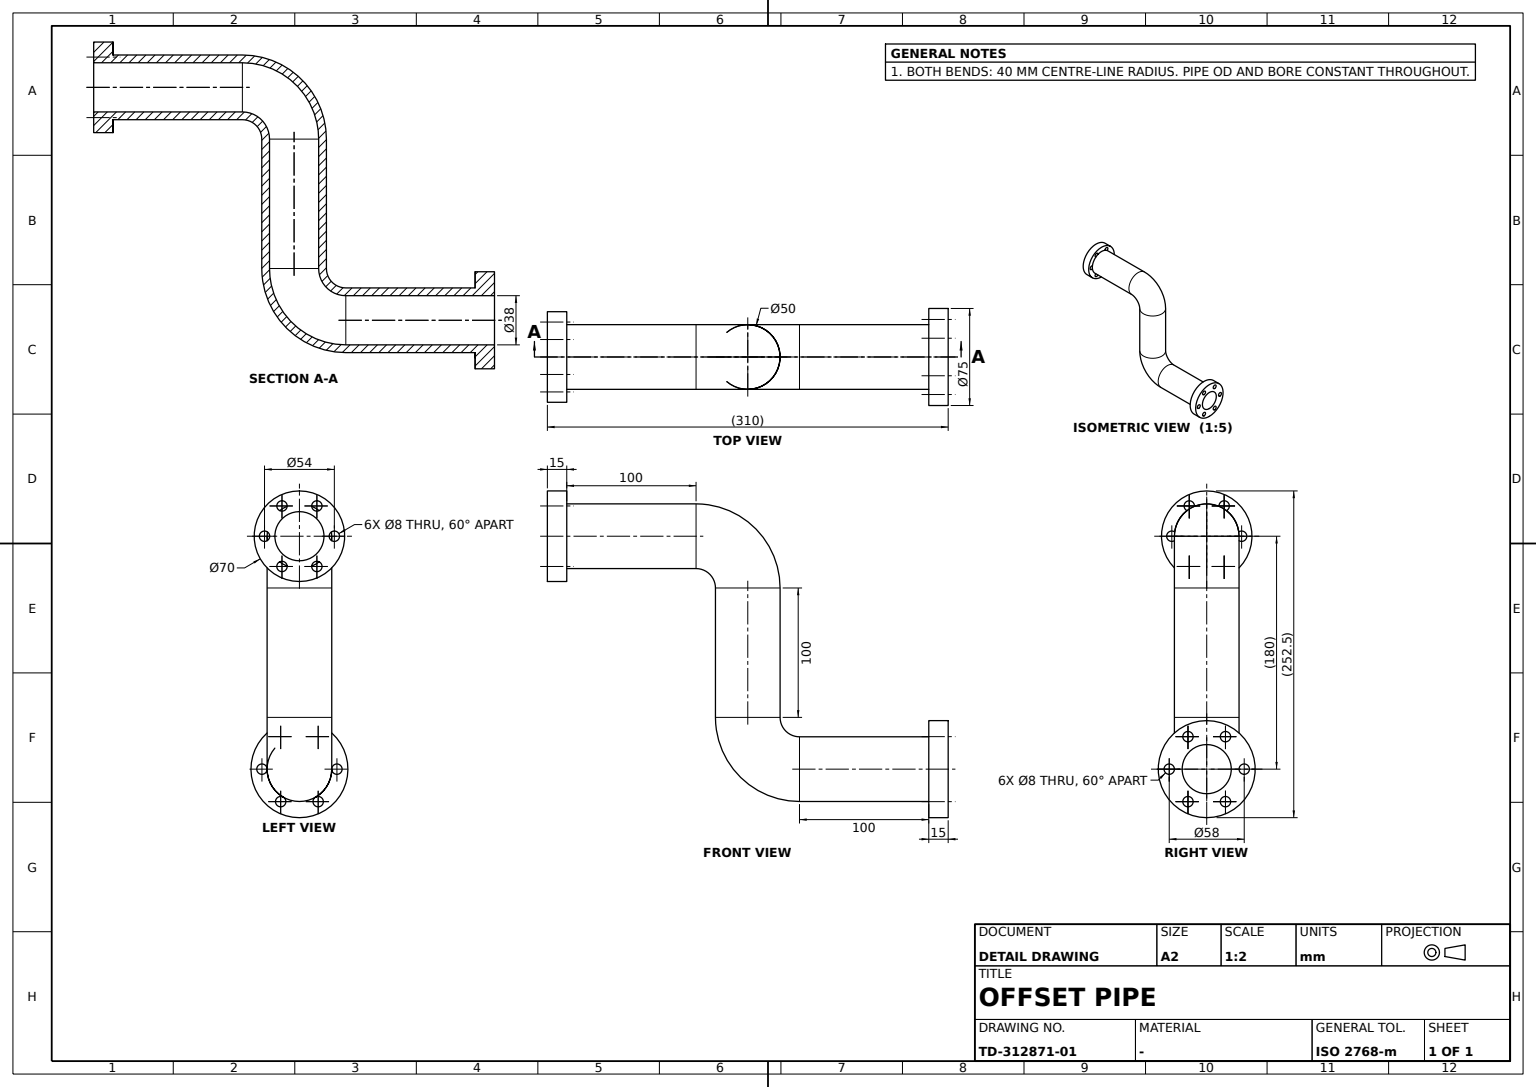
ISO-10303-21;
HEADER;
FILE_DESCRIPTION((''),'2;1');
FILE_NAME('','',(''),(''),'','','');
FILE_SCHEMA(('AUTOMOTIVE_DESIGN'));
ENDSEC;
DATA;
#1=APPLICATION_CONTEXT('');
#2=PRODUCT_CONTEXT('',#1,'mechanical');
#3=PRODUCT('','','',(#2));
#4=PRODUCT_DEFINITION_FORMATION('','',#3);
#5=PRODUCT_DEFINITION_CONTEXT('',#1,'design');
#6=PRODUCT_DEFINITION('','',#4,#5);
#7=PRODUCT_DEFINITION_SHAPE('','',#6);
#8=(LENGTH_UNIT()NAMED_UNIT(*)SI_UNIT(.MILLI.,.METRE.));
#9=(NAMED_UNIT(*)PLANE_ANGLE_UNIT()SI_UNIT($,.RADIAN.));
#10=(NAMED_UNIT(*)SI_UNIT($,.STERADIAN.)SOLID_ANGLE_UNIT());
#11=UNCERTAINTY_MEASURE_WITH_UNIT(LENGTH_MEASURE(0.005),#8,'distance_accuracy_value','');
#12=(GEOMETRIC_REPRESENTATION_CONTEXT(3)GLOBAL_UNCERTAINTY_ASSIGNED_CONTEXT((#11))GLOBAL_UNIT_ASSIGNED_CONTEXT((#8,#9,#10))REPRESENTATION_CONTEXT('',''));
#13=CARTESIAN_POINT('',(-165.,0.,40.));
#14=VERTEX_POINT('',#13);
#15=CARTESIAN_POINT('',(-140.,0.,40.));
#16=DIRECTION('',(0.,0.,-1.));
#17=DIRECTION('',(-1.,0.,0.));
#18=AXIS2_PLACEMENT_3D('',#15,#16,#17);
#19=CIRCLE('',#18,25.);
#20=EDGE_CURVE('',#14,#14,#19,.T.);
#21=ORIENTED_EDGE('',*,*,#20,.F.);
#22=EDGE_LOOP('',(#21));
#23=FACE_BOUND('',#22,.T.);
#24=CARTESIAN_POINT('',(-165.,0.,140.));
#25=VERTEX_POINT('',#24);
#26=CARTESIAN_POINT('',(-140.,0.,140.));
#27=AXIS2_PLACEMENT_3D('',#26,#16,#17);
#28=CIRCLE('',#27,25.);
#29=EDGE_CURVE('',#25,#25,#28,.T.);
#30=ORIENTED_EDGE('',*,*,#29,.T.);
#31=EDGE_LOOP('',(#30));
#32=FACE_BOUND('',#31,.T.);
#33=CARTESIAN_POINT('',(-140.,0.,90.));
#34=DIRECTION('',(0.,1.,0.));
#35=AXIS2_PLACEMENT_3D('',#33,#16,#34);
#36=CYLINDRICAL_SURFACE('',#35,25.);
#37=ADVANCED_FACE('',(#23,#32),#36,.T.);
#38=CARTESIAN_POINT('',(0.,-25.,0.));
#39=VERTEX_POINT('',#38);
#40=CARTESIAN_POINT('',(0.,-29.,0.));
#41=DIRECTION('',(1.,0.,0.));
#42=AXIS2_PLACEMENT_3D('',#40,#41,#16);
#43=CIRCLE('',#42,4.);
#44=EDGE_CURVE('',#39,#39,#43,.T.);
#45=ORIENTED_EDGE('',*,*,#44,.F.);
#46=EDGE_LOOP('',(#45));
#47=FACE_BOUND('',#46,.T.);
#48=CARTESIAN_POINT('',(15.,-29.,-4.));
#49=VERTEX_POINT('',#48);
#50=CARTESIAN_POINT('',(15.,-29.,0.));
#51=AXIS2_PLACEMENT_3D('',#50,#41,#16);
#52=CIRCLE('',#51,4.);
#53=EDGE_CURVE('',#49,#49,#52,.T.);
#54=ORIENTED_EDGE('',*,*,#53,.T.);
#55=EDGE_LOOP('',(#54));
#56=FACE_BOUND('',#55,.T.);
#57=CARTESIAN_POINT('',(7.5,-29.,0.));
#58=DIRECTION('',(0.,-1.,0.));
#59=AXIS2_PLACEMENT_3D('',#57,#41,#58);
#60=CYLINDRICAL_SURFACE('',#59,4.);
#61=ADVANCED_FACE('',(#47,#56),#60,.F.);
#62=CARTESIAN_POINT('',(15.,14.5,21.114737));
#63=VERTEX_POINT('',#62);
#64=CARTESIAN_POINT('',(15.,14.5,25.114737));
#65=AXIS2_PLACEMENT_3D('',#64,#41,#16);
#66=CIRCLE('',#65,4.);
#67=EDGE_CURVE('',#63,#63,#66,.T.);
#68=ORIENTED_EDGE('',*,*,#67,.T.);
#69=EDGE_LOOP('',(#68));
#70=FACE_BOUND('',#69,.T.);
#71=CARTESIAN_POINT('',(0.,12.5,21.650635));
#72=VERTEX_POINT('',#71);
#73=CARTESIAN_POINT('',(0.,14.5,25.114737));
#74=AXIS2_PLACEMENT_3D('',#73,#41,#16);
#75=CIRCLE('',#74,4.);
#76=EDGE_CURVE('',#72,#72,#75,.T.);
#77=ORIENTED_EDGE('',*,*,#76,.F.);
#78=EDGE_LOOP('',(#77));
#79=FACE_BOUND('',#78,.T.);
#80=CARTESIAN_POINT('',(7.5,14.5,25.114737));
#81=DIRECTION('',(0.,0.5,0.866025404));
#82=AXIS2_PLACEMENT_3D('',#80,#41,#81);
#83=CYLINDRICAL_SURFACE('',#82,4.);
#84=ADVANCED_FACE('',(#70,#79),#83,.F.);
#85=CARTESIAN_POINT('',(-180.,0.,199.));
#86=VERTEX_POINT('',#85);
#87=CARTESIAN_POINT('',(-180.,0.,180.));
#88=DIRECTION('',(0.,0.,1.));
#89=AXIS2_PLACEMENT_3D('',#87,#17,#88);
#90=CIRCLE('',#89,19.);
#91=EDGE_CURVE('',#86,#86,#90,.F.);
#92=ORIENTED_EDGE('',*,*,#91,.T.);
#93=EDGE_LOOP('',(#92));
#94=FACE_BOUND('',#93,.T.);
#95=CARTESIAN_POINT('',(-295.,0.,199.));
#96=VERTEX_POINT('',#95);
#97=CARTESIAN_POINT('',(-295.,0.,180.));
#98=AXIS2_PLACEMENT_3D('',#97,#17,#88);
#99=CIRCLE('',#98,19.);
#100=EDGE_CURVE('',#96,#96,#99,.T.);
#101=ORIENTED_EDGE('',*,*,#100,.T.);
#102=EDGE_LOOP('',(#101));
#103=FACE_BOUND('',#102,.T.);
#104=CARTESIAN_POINT('',(-287.5,0.,180.));
#105=AXIS2_PLACEMENT_3D('',#104,#17,#58);
#106=CYLINDRICAL_SURFACE('',#105,19.);
#107=ADVANCED_FACE('',(#94,#103),#106,.F.);
#108=CARTESIAN_POINT('',(-280.,24.777778,176.674082));
#109=VERTEX_POINT('',#108);
#110=CARTESIAN_POINT('',(-280.,24.777778,183.325918));
#111=VERTEX_POINT('',#110);
#112=CARTESIAN_POINT('',(-280.,0.,180.));
#113=AXIS2_PLACEMENT_3D('',#112,#41,#16);
#114=CIRCLE('',#113,25.);
#115=EDGE_CURVE('',#109,#111,#114,.T.);
#116=ORIENTED_EDGE('',*,*,#115,.F.);
#117=CARTESIAN_POINT('',(-280.,27.,180.));
#118=AXIS2_PLACEMENT_3D('',#117,#41,#16);
#119=CIRCLE('',#118,4.);
#120=EDGE_CURVE('',#109,#111,#119,.F.);
#121=ORIENTED_EDGE('',*,*,#120,.T.);
#122=EDGE_LOOP('',(#116,#121));
#123=FACE_BOUND('',#122,.T.);
#124=AXIS2_PLACEMENT_3D('',#112,#41,#34);
#125=PLANE('',#124);
#126=ADVANCED_FACE('',(#123),#125,.F.);
#127=CARTESIAN_POINT('',(-100.,0.,-19.));
#128=VERTEX_POINT('',#127);
#129=CARTESIAN_POINT('',(-100.,0.,0.));
#130=AXIS2_PLACEMENT_3D('',#129,#41,#16);
#131=CIRCLE('',#130,19.);
#132=EDGE_CURVE('',#128,#128,#131,.T.);
#133=ORIENTED_EDGE('',*,*,#132,.F.);
#134=EDGE_LOOP('',(#133));
#135=FACE_BOUND('',#134,.T.);
#136=CARTESIAN_POINT('',(15.,0.,-19.));
#137=VERTEX_POINT('',#136);
#138=CARTESIAN_POINT('',(15.,0.,0.));
#139=AXIS2_PLACEMENT_3D('',#138,#41,#16);
#140=CIRCLE('',#139,19.);
#141=EDGE_CURVE('',#137,#137,#140,.T.);
#142=ORIENTED_EDGE('',*,*,#141,.T.);
#143=EDGE_LOOP('',(#142));
#144=FACE_BOUND('',#143,.T.);
#145=CARTESIAN_POINT('',(-50.,0.,0.));
#146=AXIS2_PLACEMENT_3D('',#145,#41,#34);
#147=CYLINDRICAL_SURFACE('',#146,19.);
#148=ADVANCED_FACE('',(#135,#144),#147,.F.);
#149=CARTESIAN_POINT('',(0.,-12.5,21.650635));
#150=VERTEX_POINT('',#149);
#151=CARTESIAN_POINT('',(0.,0.,0.));
#152=AXIS2_PLACEMENT_3D('',#151,#41,#16);
#153=CIRCLE('',#152,25.);
#154=EDGE_CURVE('',#72,#150,#153,.T.);
#155=ORIENTED_EDGE('',*,*,#154,.T.);
#156=CARTESIAN_POINT('',(0.,-14.5,25.114737));
#157=AXIS2_PLACEMENT_3D('',#156,#41,#16);
#158=CIRCLE('',#157,4.);
#159=EDGE_CURVE('',#150,#150,#158,.T.);
#160=ORIENTED_EDGE('',*,*,#159,.T.);
#161=EDGE_CURVE('',#150,#39,#153,.T.);
#162=ORIENTED_EDGE('',*,*,#161,.T.);
#163=ORIENTED_EDGE('',*,*,#44,.T.);
#164=CARTESIAN_POINT('',(0.,-12.5,-21.650635));
#165=VERTEX_POINT('',#164);
#166=EDGE_CURVE('',#39,#165,#153,.T.);
#167=ORIENTED_EDGE('',*,*,#166,.T.);
#168=CARTESIAN_POINT('',(0.,-14.5,-25.114737));
#169=AXIS2_PLACEMENT_3D('',#168,#41,#16);
#170=CIRCLE('',#169,4.);
#171=EDGE_CURVE('',#165,#165,#170,.T.);
#172=ORIENTED_EDGE('',*,*,#171,.T.);
#173=CARTESIAN_POINT('',(0.,12.5,-21.650635));
#174=VERTEX_POINT('',#173);
#175=EDGE_CURVE('',#165,#174,#153,.T.);
#176=ORIENTED_EDGE('',*,*,#175,.T.);
#177=CARTESIAN_POINT('',(0.,14.5,-25.114737));
#178=AXIS2_PLACEMENT_3D('',#177,#41,#16);
#179=CIRCLE('',#178,4.);
#180=EDGE_CURVE('',#174,#174,#179,.T.);
#181=ORIENTED_EDGE('',*,*,#180,.T.);
#182=CARTESIAN_POINT('',(0.,25.,0.));
#183=VERTEX_POINT('',#182);
#184=EDGE_CURVE('',#174,#183,#153,.T.);
#185=ORIENTED_EDGE('',*,*,#184,.T.);
#186=CARTESIAN_POINT('',(0.,29.,0.));
#187=AXIS2_PLACEMENT_3D('',#186,#41,#16);
#188=CIRCLE('',#187,4.);
#189=EDGE_CURVE('',#183,#183,#188,.T.);
#190=ORIENTED_EDGE('',*,*,#189,.T.);
#191=EDGE_CURVE('',#183,#72,#153,.T.);
#192=ORIENTED_EDGE('',*,*,#191,.T.);
#193=ORIENTED_EDGE('',*,*,#76,.T.);
#194=EDGE_LOOP('',(#155,#160,#162,#163,#167,#172,#176,#181,#185,#190,#192,#193));
#195=FACE_BOUND('',#194,.T.);
#196=CARTESIAN_POINT('',(0.,0.,-37.5));
#197=VERTEX_POINT('',#196);
#198=CIRCLE('',#152,37.5);
#199=EDGE_CURVE('',#197,#197,#198,.T.);
#200=ORIENTED_EDGE('',*,*,#199,.F.);
#201=EDGE_LOOP('',(#200));
#202=FACE_BOUND('',#201,.T.);
#203=AXIS2_PLACEMENT_3D('',#151,#41,#34);
#204=PLANE('',#203);
#205=ADVANCED_FACE('',(#195,#202),#204,.F.);
#206=CARTESIAN_POINT('',(-159.,0.,140.));
#207=VERTEX_POINT('',#206);
#208=CIRCLE('',#27,19.);
#209=EDGE_CURVE('',#207,#207,#208,.T.);
#210=ORIENTED_EDGE('',*,*,#209,.T.);
#211=EDGE_LOOP('',(#210));
#212=FACE_BOUND('',#211,.T.);
#213=ORIENTED_EDGE('',*,*,#91,.F.);
#214=EDGE_LOOP('',(#213));
#215=FACE_BOUND('',#214,.T.);
#216=CARTESIAN_POINT('',(-180.,0.,140.));
#217=AXIS2_PLACEMENT_3D('',#216,#34,#88);
#218=TOROIDAL_SURFACE('',#217,40.,19.);
#219=ADVANCED_FACE('',(#212,#215),#218,.F.);
#220=ORIENTED_EDGE('',*,*,#159,.F.);
#221=EDGE_LOOP('',(#220));
#222=FACE_BOUND('',#221,.T.);
#223=CARTESIAN_POINT('',(15.,-14.5,21.114737));
#224=VERTEX_POINT('',#223);
#225=CARTESIAN_POINT('',(15.,-14.5,25.114737));
#226=AXIS2_PLACEMENT_3D('',#225,#41,#16);
#227=CIRCLE('',#226,4.);
#228=EDGE_CURVE('',#224,#224,#227,.T.);
#229=ORIENTED_EDGE('',*,*,#228,.T.);
#230=EDGE_LOOP('',(#229));
#231=FACE_BOUND('',#230,.T.);
#232=CARTESIAN_POINT('',(7.5,-14.5,25.114737));
#233=DIRECTION('',(0.,-0.5,0.866025404));
#234=AXIS2_PLACEMENT_3D('',#232,#41,#233);
#235=CYLINDRICAL_SURFACE('',#234,4.);
#236=ADVANCED_FACE('',(#222,#231),#235,.F.);
#237=CARTESIAN_POINT('',(-280.,-24.777778,183.325918));
#238=VERTEX_POINT('',#237);
#239=CARTESIAN_POINT('',(-280.,-24.777778,176.674082));
#240=VERTEX_POINT('',#239);
#241=CARTESIAN_POINT('',(-280.,-27.,180.));
#242=AXIS2_PLACEMENT_3D('',#241,#41,#16);
#243=CIRCLE('',#242,4.);
#244=EDGE_CURVE('',#238,#240,#243,.F.);
#245=ORIENTED_EDGE('',*,*,#244,.T.);
#246=EDGE_CURVE('',#238,#240,#114,.T.);
#247=ORIENTED_EDGE('',*,*,#246,.F.);
#248=EDGE_LOOP('',(#245,#247));
#249=FACE_BOUND('',#248,.T.);
#250=ADVANCED_FACE('',(#249),#125,.F.);
#251=ORIENTED_EDGE('',*,*,#180,.F.);
#252=EDGE_LOOP('',(#251));
#253=FACE_BOUND('',#252,.T.);
#254=CARTESIAN_POINT('',(15.,14.5,-29.114737));
#255=VERTEX_POINT('',#254);
#256=CARTESIAN_POINT('',(15.,14.5,-25.114737));
#257=AXIS2_PLACEMENT_3D('',#256,#41,#16);
#258=CIRCLE('',#257,4.);
#259=EDGE_CURVE('',#255,#255,#258,.T.);
#260=ORIENTED_EDGE('',*,*,#259,.T.);
#261=EDGE_LOOP('',(#260));
#262=FACE_BOUND('',#261,.T.);
#263=CARTESIAN_POINT('',(7.5,14.5,-25.114737));
#264=DIRECTION('',(0.,0.5,-0.866025404));
#265=AXIS2_PLACEMENT_3D('',#263,#41,#264);
#266=CYLINDRICAL_SURFACE('',#265,4.);
#267=ADVANCED_FACE('',(#253,#262),#266,.F.);
#268=CARTESIAN_POINT('',(-295.,0.,215.));
#269=VERTEX_POINT('',#268);
#270=CIRCLE('',#98,35.);
#271=EDGE_CURVE('',#269,#269,#270,.T.);
#272=ORIENTED_EDGE('',*,*,#271,.F.);
#273=EDGE_LOOP('',(#272));
#274=FACE_BOUND('',#273,.T.);
#275=CARTESIAN_POINT('',(-280.,0.,145.));
#276=VERTEX_POINT('',#275);
#277=CIRCLE('',#113,35.);
#278=EDGE_CURVE('',#276,#276,#277,.F.);
#279=ORIENTED_EDGE('',*,*,#278,.T.);
#280=EDGE_LOOP('',(#279));
#281=FACE_BOUND('',#280,.T.);
#282=CYLINDRICAL_SURFACE('',#105,35.);
#283=ADVANCED_FACE('',(#274,#281),#282,.T.);
#284=CARTESIAN_POINT('',(-280.,-9.50856,203.121144));
#285=VERTEX_POINT('',#284);
#286=CARTESIAN_POINT('',(-280.,-15.269218,199.795226));
#287=VERTEX_POINT('',#286);
#288=CARTESIAN_POINT('',(-280.,-13.5,203.382686));
#289=AXIS2_PLACEMENT_3D('',#288,#41,#16);
#290=CIRCLE('',#289,4.);
#291=EDGE_CURVE('',#285,#287,#290,.F.);
#292=ORIENTED_EDGE('',*,*,#291,.T.);
#293=EDGE_CURVE('',#285,#287,#114,.T.);
#294=ORIENTED_EDGE('',*,*,#293,.F.);
#295=EDGE_LOOP('',(#292,#294));
#296=FACE_BOUND('',#295,.T.);
#297=ADVANCED_FACE('',(#296),#125,.F.);
#298=CARTESIAN_POINT('',(15.,-14.5,-29.114737));
#299=VERTEX_POINT('',#298);
#300=CARTESIAN_POINT('',(15.,-14.5,-25.114737));
#301=AXIS2_PLACEMENT_3D('',#300,#41,#16);
#302=CIRCLE('',#301,4.);
#303=EDGE_CURVE('',#299,#299,#302,.T.);
#304=ORIENTED_EDGE('',*,*,#303,.F.);
#305=EDGE_LOOP('',(#304));
#306=FACE_BOUND('',#305,.T.);
#307=ORIENTED_EDGE('',*,*,#259,.F.);
#308=EDGE_LOOP('',(#307));
#309=FACE_BOUND('',#308,.T.);
#310=ORIENTED_EDGE('',*,*,#141,.F.);
#311=EDGE_LOOP('',(#310));
#312=FACE_BOUND('',#311,.T.);
#313=ORIENTED_EDGE('',*,*,#53,.F.);
#314=EDGE_LOOP('',(#313));
#315=FACE_BOUND('',#314,.T.);
#316=CARTESIAN_POINT('',(15.,0.,-37.5));
#317=VERTEX_POINT('',#316);
#318=CIRCLE('',#139,37.5);
#319=EDGE_CURVE('',#317,#317,#318,.T.);
#320=ORIENTED_EDGE('',*,*,#319,.T.);
#321=EDGE_LOOP('',(#320));
#322=FACE_BOUND('',#321,.T.);
#323=CARTESIAN_POINT('',(15.,29.,-4.));
#324=VERTEX_POINT('',#323);
#325=CARTESIAN_POINT('',(15.,29.,0.));
#326=AXIS2_PLACEMENT_3D('',#325,#41,#16);
#327=CIRCLE('',#326,4.);
#328=EDGE_CURVE('',#324,#324,#327,.T.);
#329=ORIENTED_EDGE('',*,*,#328,.F.);
#330=EDGE_LOOP('',(#329));
#331=FACE_BOUND('',#330,.T.);
#332=ORIENTED_EDGE('',*,*,#228,.F.);
#333=EDGE_LOOP('',(#332));
#334=FACE_BOUND('',#333,.T.);
#335=ORIENTED_EDGE('',*,*,#67,.F.);
#336=EDGE_LOOP('',(#335));
#337=FACE_BOUND('',#336,.T.);
#338=AXIS2_PLACEMENT_3D('',#138,#41,#34);
#339=PLANE('',#338);
#340=ADVANCED_FACE('',(#306,#309,#312,#315,#322,#331,#334,#337),#339,.T.);
#341=CARTESIAN_POINT('',(-280.,9.50856,203.121144));
#342=VERTEX_POINT('',#341);
#343=CARTESIAN_POINT('',(-280.,15.269218,199.795226));
#344=VERTEX_POINT('',#343);
#345=CARTESIAN_POINT('',(-280.,13.5,203.382686));
#346=AXIS2_PLACEMENT_3D('',#345,#41,#16);
#347=CIRCLE('',#346,4.);
#348=EDGE_CURVE('',#342,#344,#347,.F.);
#349=ORIENTED_EDGE('',*,*,#348,.F.);
#350=EDGE_CURVE('',#344,#342,#347,.F.);
#351=ORIENTED_EDGE('',*,*,#350,.F.);
#352=EDGE_LOOP('',(#349,#351));
#353=FACE_BOUND('',#352,.T.);
#354=CARTESIAN_POINT('',(-295.,13.5,207.382686));
#355=VERTEX_POINT('',#354);
#356=CARTESIAN_POINT('',(-295.,13.5,203.382686));
#357=AXIS2_PLACEMENT_3D('',#356,#17,#88);
#358=CIRCLE('',#357,4.);
#359=EDGE_CURVE('',#355,#355,#358,.T.);
#360=ORIENTED_EDGE('',*,*,#359,.T.);
#361=EDGE_LOOP('',(#360));
#362=FACE_BOUND('',#361,.T.);
#363=CARTESIAN_POINT('',(-287.5,13.5,203.382686));
#364=AXIS2_PLACEMENT_3D('',#363,#17,#81);
#365=CYLINDRICAL_SURFACE('',#364,4.);
#366=ADVANCED_FACE('',(#353,#362),#365,.F.);
#367=CARTESIAN_POINT('',(-280.,-15.269218,160.204774));
#368=VERTEX_POINT('',#367);
#369=CARTESIAN_POINT('',(-280.,-9.50856,156.878856));
#370=VERTEX_POINT('',#369);
#371=CARTESIAN_POINT('',(-280.,-13.5,156.617314));
#372=AXIS2_PLACEMENT_3D('',#371,#41,#16);
#373=CIRCLE('',#372,4.);
#374=EDGE_CURVE('',#368,#370,#373,.F.);
#375=ORIENTED_EDGE('',*,*,#374,.T.);
#376=EDGE_CURVE('',#368,#370,#114,.T.);
#377=ORIENTED_EDGE('',*,*,#376,.F.);
#378=EDGE_LOOP('',(#375,#377));
#379=FACE_BOUND('',#378,.T.);
#380=ADVANCED_FACE('',(#379),#125,.F.);
#381=CARTESIAN_POINT('',(-295.,-13.5,160.617314));
#382=VERTEX_POINT('',#381);
#383=CARTESIAN_POINT('',(-295.,-13.5,156.617314));
#384=AXIS2_PLACEMENT_3D('',#383,#17,#88);
#385=CIRCLE('',#384,4.);
#386=EDGE_CURVE('',#382,#382,#385,.T.);
#387=ORIENTED_EDGE('',*,*,#386,.T.);
#388=EDGE_LOOP('',(#387));
#389=FACE_BOUND('',#388,.T.);
#390=EDGE_CURVE('',#370,#368,#373,.F.);
#391=ORIENTED_EDGE('',*,*,#390,.F.);
#392=ORIENTED_EDGE('',*,*,#374,.F.);
#393=EDGE_LOOP('',(#391,#392));
#394=FACE_BOUND('',#393,.T.);
#395=CARTESIAN_POINT('',(-287.5,-13.5,156.617314));
#396=DIRECTION('',(0.,-0.5,-0.866025404));
#397=AXIS2_PLACEMENT_3D('',#395,#17,#396);
#398=CYLINDRICAL_SURFACE('',#397,4.);
#399=ADVANCED_FACE('',(#389,#394),#398,.F.);
#400=CARTESIAN_POINT('',(-159.,0.,40.));
#401=VERTEX_POINT('',#400);
#402=CIRCLE('',#18,19.);
#403=EDGE_CURVE('',#401,#401,#402,.T.);
#404=ORIENTED_EDGE('',*,*,#403,.F.);
#405=EDGE_LOOP('',(#404));
#406=FACE_BOUND('',#405,.T.);
#407=ORIENTED_EDGE('',*,*,#132,.T.);
#408=EDGE_LOOP('',(#407));
#409=FACE_BOUND('',#408,.T.);
#410=CARTESIAN_POINT('',(-100.,0.,40.));
#411=AXIS2_PLACEMENT_3D('',#410,#34,#16);
#412=TOROIDAL_SURFACE('',#411,40.,19.);
#413=ADVANCED_FACE('',(#406,#409),#412,.F.);
#414=EDGE_CURVE('',#287,#238,#114,.T.);
#415=ORIENTED_EDGE('',*,*,#414,.F.);
#416=EDGE_CURVE('',#287,#285,#290,.F.);
#417=ORIENTED_EDGE('',*,*,#416,.T.);
#418=EDGE_CURVE('',#342,#285,#114,.T.);
#419=ORIENTED_EDGE('',*,*,#418,.F.);
#420=ORIENTED_EDGE('',*,*,#348,.T.);
#421=EDGE_CURVE('',#111,#344,#114,.T.);
#422=ORIENTED_EDGE('',*,*,#421,.F.);
#423=EDGE_CURVE('',#111,#109,#119,.F.);
#424=ORIENTED_EDGE('',*,*,#423,.T.);
#425=CARTESIAN_POINT('',(-280.,15.269218,160.204774));
#426=VERTEX_POINT('',#425);
#427=EDGE_CURVE('',#426,#109,#114,.T.);
#428=ORIENTED_EDGE('',*,*,#427,.F.);
#429=CARTESIAN_POINT('',(-280.,9.50856,156.878856));
#430=VERTEX_POINT('',#429);
#431=CARTESIAN_POINT('',(-280.,13.5,156.617314));
#432=AXIS2_PLACEMENT_3D('',#431,#41,#16);
#433=CIRCLE('',#432,4.);
#434=EDGE_CURVE('',#426,#430,#433,.F.);
#435=ORIENTED_EDGE('',*,*,#434,.T.);
#436=EDGE_CURVE('',#370,#430,#114,.T.);
#437=ORIENTED_EDGE('',*,*,#436,.F.);
#438=ORIENTED_EDGE('',*,*,#390,.T.);
#439=EDGE_CURVE('',#240,#368,#114,.T.);
#440=ORIENTED_EDGE('',*,*,#439,.F.);
#441=EDGE_CURVE('',#240,#238,#243,.F.);
#442=ORIENTED_EDGE('',*,*,#441,.T.);
#443=EDGE_LOOP('',(#415,#417,#419,#420,#422,#424,#428,#435,#437,#438,#440,#442));
#444=FACE_BOUND('',#443,.T.);
#445=ORIENTED_EDGE('',*,*,#278,.F.);
#446=EDGE_LOOP('',(#445));
#447=FACE_BOUND('',#446,.T.);
#448=ADVANCED_FACE('',(#444,#447),#125,.T.);
#449=ORIENTED_EDGE('',*,*,#20,.T.);
#450=EDGE_LOOP('',(#449));
#451=FACE_BOUND('',#450,.T.);
#452=CARTESIAN_POINT('',(-100.,0.,-25.));
#453=VERTEX_POINT('',#452);
#454=CIRCLE('',#130,25.);
#455=EDGE_CURVE('',#453,#453,#454,.T.);
#456=ORIENTED_EDGE('',*,*,#455,.F.);
#457=EDGE_LOOP('',(#456));
#458=FACE_BOUND('',#457,.T.);
#459=TOROIDAL_SURFACE('',#411,40.,25.);
#460=ADVANCED_FACE('',(#451,#458),#459,.T.);
#461=ORIENTED_EDGE('',*,*,#184,.F.);
#462=ORIENTED_EDGE('',*,*,#175,.F.);
#463=ORIENTED_EDGE('',*,*,#166,.F.);
#464=ORIENTED_EDGE('',*,*,#161,.F.);
#465=ORIENTED_EDGE('',*,*,#154,.F.);
#466=ORIENTED_EDGE('',*,*,#191,.F.);
#467=EDGE_LOOP('',(#461,#462,#463,#464,#465,#466));
#468=FACE_BOUND('',#467,.T.);
#469=ORIENTED_EDGE('',*,*,#455,.T.);
#470=EDGE_LOOP('',(#469));
#471=FACE_BOUND('',#470,.T.);
#472=CYLINDRICAL_SURFACE('',#146,25.);
#473=ADVANCED_FACE('',(#468,#471),#472,.T.);
#474=CARTESIAN_POINT('',(-295.,-27.,184.));
#475=VERTEX_POINT('',#474);
#476=CARTESIAN_POINT('',(-295.,-27.,180.));
#477=AXIS2_PLACEMENT_3D('',#476,#17,#88);
#478=CIRCLE('',#477,4.);
#479=EDGE_CURVE('',#475,#475,#478,.T.);
#480=ORIENTED_EDGE('',*,*,#479,.T.);
#481=EDGE_LOOP('',(#480));
#482=FACE_BOUND('',#481,.T.);
#483=ORIENTED_EDGE('',*,*,#244,.F.);
#484=ORIENTED_EDGE('',*,*,#441,.F.);
#485=EDGE_LOOP('',(#483,#484));
#486=FACE_BOUND('',#485,.T.);
#487=CARTESIAN_POINT('',(-287.5,-27.,180.));
#488=AXIS2_PLACEMENT_3D('',#487,#17,#58);
#489=CYLINDRICAL_SURFACE('',#488,4.);
#490=ADVANCED_FACE('',(#482,#486),#489,.F.);
#491=ORIENTED_EDGE('',*,*,#209,.F.);
#492=EDGE_LOOP('',(#491));
#493=FACE_BOUND('',#492,.T.);
#494=ORIENTED_EDGE('',*,*,#403,.T.);
#495=EDGE_LOOP('',(#494));
#496=FACE_BOUND('',#495,.T.);
#497=CYLINDRICAL_SURFACE('',#35,19.);
#498=ADVANCED_FACE('',(#493,#496),#497,.F.);
#499=EDGE_CURVE('',#430,#426,#114,.T.);
#500=ORIENTED_EDGE('',*,*,#499,.F.);
#501=EDGE_CURVE('',#430,#426,#433,.F.);
#502=ORIENTED_EDGE('',*,*,#501,.T.);
#503=EDGE_LOOP('',(#500,#502));
#504=FACE_BOUND('',#503,.T.);
#505=ADVANCED_FACE('',(#504),#125,.F.);
#506=ORIENTED_EDGE('',*,*,#303,.T.);
#507=EDGE_LOOP('',(#506));
#508=FACE_BOUND('',#507,.T.);
#509=ORIENTED_EDGE('',*,*,#171,.F.);
#510=EDGE_LOOP('',(#509));
#511=FACE_BOUND('',#510,.T.);
#512=CARTESIAN_POINT('',(7.5,-14.5,-25.114737));
#513=AXIS2_PLACEMENT_3D('',#512,#41,#396);
#514=CYLINDRICAL_SURFACE('',#513,4.);
#515=ADVANCED_FACE('',(#508,#511),#514,.F.);
#516=EDGE_CURVE('',#344,#342,#114,.T.);
#517=ORIENTED_EDGE('',*,*,#516,.T.);
#518=ORIENTED_EDGE('',*,*,#418,.T.);
#519=ORIENTED_EDGE('',*,*,#293,.T.);
#520=ORIENTED_EDGE('',*,*,#414,.T.);
#521=ORIENTED_EDGE('',*,*,#246,.T.);
#522=ORIENTED_EDGE('',*,*,#439,.T.);
#523=ORIENTED_EDGE('',*,*,#376,.T.);
#524=ORIENTED_EDGE('',*,*,#436,.T.);
#525=ORIENTED_EDGE('',*,*,#499,.T.);
#526=ORIENTED_EDGE('',*,*,#427,.T.);
#527=ORIENTED_EDGE('',*,*,#115,.T.);
#528=ORIENTED_EDGE('',*,*,#421,.T.);
#529=EDGE_LOOP('',(#517,#518,#519,#520,#521,#522,#523,#524,#525,#526,#527,#528));
#530=FACE_BOUND('',#529,.T.);
#531=CARTESIAN_POINT('',(-180.,0.,155.));
#532=VERTEX_POINT('',#531);
#533=AXIS2_PLACEMENT_3D('',#87,#41,#16);
#534=CIRCLE('',#533,25.);
#535=EDGE_CURVE('',#532,#532,#534,.T.);
#536=ORIENTED_EDGE('',*,*,#535,.F.);
#537=EDGE_LOOP('',(#536));
#538=FACE_BOUND('',#537,.T.);
#539=CARTESIAN_POINT('',(-230.,0.,180.));
#540=AXIS2_PLACEMENT_3D('',#539,#41,#34);
#541=CYLINDRICAL_SURFACE('',#540,25.);
#542=ADVANCED_FACE('',(#530,#538),#541,.T.);
#543=ORIENTED_EDGE('',*,*,#479,.F.);
#544=EDGE_LOOP('',(#543));
#545=FACE_BOUND('',#544,.T.);
#546=ORIENTED_EDGE('',*,*,#271,.T.);
#547=EDGE_LOOP('',(#546));
#548=FACE_BOUND('',#547,.T.);
#549=CARTESIAN_POINT('',(-295.,27.,184.));
#550=VERTEX_POINT('',#549);
#551=CARTESIAN_POINT('',(-295.,27.,180.));
#552=AXIS2_PLACEMENT_3D('',#551,#17,#88);
#553=CIRCLE('',#552,4.);
#554=EDGE_CURVE('',#550,#550,#553,.T.);
#555=ORIENTED_EDGE('',*,*,#554,.F.);
#556=EDGE_LOOP('',(#555));
#557=FACE_BOUND('',#556,.T.);
#558=ORIENTED_EDGE('',*,*,#359,.F.);
#559=EDGE_LOOP('',(#558));
#560=FACE_BOUND('',#559,.T.);
#561=ORIENTED_EDGE('',*,*,#100,.F.);
#562=EDGE_LOOP('',(#561));
#563=FACE_BOUND('',#562,.T.);
#564=ORIENTED_EDGE('',*,*,#386,.F.);
#565=EDGE_LOOP('',(#564));
#566=FACE_BOUND('',#565,.T.);
#567=CARTESIAN_POINT('',(-295.,-13.5,207.382686));
#568=VERTEX_POINT('',#567);
#569=CARTESIAN_POINT('',(-295.,-13.5,203.382686));
#570=AXIS2_PLACEMENT_3D('',#569,#17,#88);
#571=CIRCLE('',#570,4.);
#572=EDGE_CURVE('',#568,#568,#571,.T.);
#573=ORIENTED_EDGE('',*,*,#572,.F.);
#574=EDGE_LOOP('',(#573));
#575=FACE_BOUND('',#574,.T.);
#576=CARTESIAN_POINT('',(-295.,13.5,160.617314));
#577=VERTEX_POINT('',#576);
#578=CARTESIAN_POINT('',(-295.,13.5,156.617314));
#579=AXIS2_PLACEMENT_3D('',#578,#17,#88);
#580=CIRCLE('',#579,4.);
#581=EDGE_CURVE('',#577,#577,#580,.T.);
#582=ORIENTED_EDGE('',*,*,#581,.F.);
#583=EDGE_LOOP('',(#582));
#584=FACE_BOUND('',#583,.T.);
#585=CARTESIAN_POINT('',(-295.,0.,0.));
#586=AXIS2_PLACEMENT_3D('',#585,#17,#58);
#587=PLANE('',#586);
#588=ADVANCED_FACE('',(#545,#548,#557,#560,#563,#566,#575,#584),#587,.T.);
#589=ORIENTED_EDGE('',*,*,#581,.T.);
#590=EDGE_LOOP('',(#589));
#591=FACE_BOUND('',#590,.T.);
#592=ORIENTED_EDGE('',*,*,#434,.F.);
#593=ORIENTED_EDGE('',*,*,#501,.F.);
#594=EDGE_LOOP('',(#592,#593));
#595=FACE_BOUND('',#594,.T.);
#596=CARTESIAN_POINT('',(-287.5,13.5,156.617314));
#597=AXIS2_PLACEMENT_3D('',#596,#17,#264);
#598=CYLINDRICAL_SURFACE('',#597,4.);
#599=ADVANCED_FACE('',(#591,#595),#598,.F.);
#600=ORIENTED_EDGE('',*,*,#319,.F.);
#601=EDGE_LOOP('',(#600));
#602=FACE_BOUND('',#601,.T.);
#603=ORIENTED_EDGE('',*,*,#199,.T.);
#604=EDGE_LOOP('',(#603));
#605=FACE_BOUND('',#604,.T.);
#606=CARTESIAN_POINT('',(7.5,0.,0.));
#607=AXIS2_PLACEMENT_3D('',#606,#41,#34);
#608=CYLINDRICAL_SURFACE('',#607,37.5);
#609=ADVANCED_FACE('',(#602,#605),#608,.T.);
#610=ORIENTED_EDGE('',*,*,#416,.F.);
#611=ORIENTED_EDGE('',*,*,#291,.F.);
#612=EDGE_LOOP('',(#610,#611));
#613=FACE_BOUND('',#612,.T.);
#614=ORIENTED_EDGE('',*,*,#572,.T.);
#615=EDGE_LOOP('',(#614));
#616=FACE_BOUND('',#615,.T.);
#617=CARTESIAN_POINT('',(-287.5,-13.5,203.382686));
#618=AXIS2_PLACEMENT_3D('',#617,#17,#233);
#619=CYLINDRICAL_SURFACE('',#618,4.);
#620=ADVANCED_FACE('',(#613,#616),#619,.F.);
#621=ORIENTED_EDGE('',*,*,#516,.F.);
#622=ORIENTED_EDGE('',*,*,#350,.T.);
#623=EDGE_LOOP('',(#621,#622));
#624=FACE_BOUND('',#623,.T.);
#625=ADVANCED_FACE('',(#624),#125,.F.);
#626=ORIENTED_EDGE('',*,*,#189,.F.);
#627=EDGE_LOOP('',(#626));
#628=FACE_BOUND('',#627,.T.);
#629=ORIENTED_EDGE('',*,*,#328,.T.);
#630=EDGE_LOOP('',(#629));
#631=FACE_BOUND('',#630,.T.);
#632=CARTESIAN_POINT('',(7.5,29.,0.));
#633=AXIS2_PLACEMENT_3D('',#632,#41,#34);
#634=CYLINDRICAL_SURFACE('',#633,4.);
#635=ADVANCED_FACE('',(#628,#631),#634,.F.);
#636=ORIENTED_EDGE('',*,*,#120,.F.);
#637=ORIENTED_EDGE('',*,*,#423,.F.);
#638=EDGE_LOOP('',(#636,#637));
#639=FACE_BOUND('',#638,.T.);
#640=ORIENTED_EDGE('',*,*,#554,.T.);
#641=EDGE_LOOP('',(#640));
#642=FACE_BOUND('',#641,.T.);
#643=CARTESIAN_POINT('',(-287.5,27.,180.));
#644=AXIS2_PLACEMENT_3D('',#643,#17,#34);
#645=CYLINDRICAL_SURFACE('',#644,4.);
#646=ADVANCED_FACE('',(#639,#642),#645,.F.);
#647=ORIENTED_EDGE('',*,*,#535,.T.);
#648=EDGE_LOOP('',(#647));
#649=FACE_BOUND('',#648,.T.);
#650=ORIENTED_EDGE('',*,*,#29,.F.);
#651=EDGE_LOOP('',(#650));
#652=FACE_BOUND('',#651,.T.);
#653=TOROIDAL_SURFACE('',#217,40.,25.);
#654=ADVANCED_FACE('',(#649,#652),#653,.T.);
#655=CLOSED_SHELL('',(#37,#61,#84,#107,#126,#148,#205,#219,#236,#250,#267,#283,#297,#340,#366,#380,#399,#413,#448,#460,#473,#490,#498,#505,#515,#542,#588,#599,#609,#620,#625,#635,#646,#654));
#656=MANIFOLD_SOLID_BREP('',#655);
#657=ADVANCED_BREP_SHAPE_REPRESENTATION('',(#656),#12);
#658=SHAPE_DEFINITION_REPRESENTATION(#7,#657);
ENDSEC;
END-ISO-10303-21;
